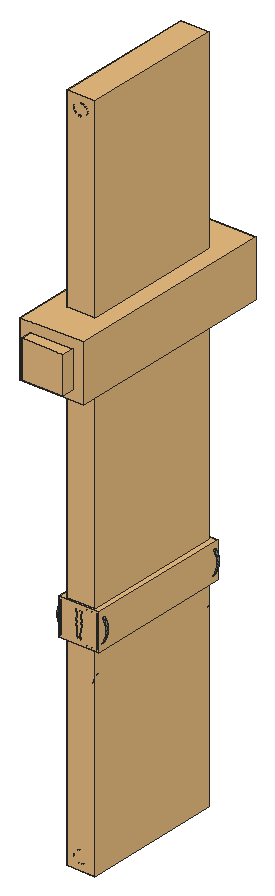
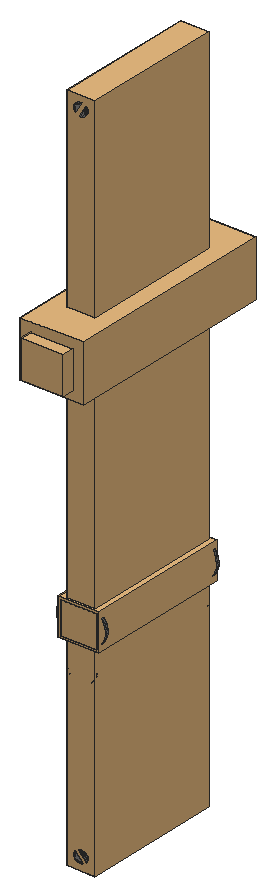
# SketchUp Ruby script. Lengths in inches.
U = 1.inch
M = Sketchup.active_model
def pt(a) = Geom::Point3d.new(a.map { |v| v * U })
def face(e, loops, mat)
  f = e.add_face(loops[0].map { |a| pt(a) })
  loops[1..].each { |l| e.add_face(l.map { |a| pt(a) }).erase! }
  f.material = f.back_material = mat if mat
  f
end
# faces: each face lists its corners as indices into pts; further lists are holes
def faces(e, pts, list, mat = nil) = list.each { |f| face(e, (f[0].is_a?(Array) ? f : [f]).map { |l| l.map { |i| pts[i] } }, mat) }
# xy, xz, yz: faces in a plane at the given z, y or x. An outline is a flat list of corners, or four numbers for a rectangle; further outlines are holes
def ring(l) = l.size == 4 ? [[l[0], l[1]], [l[2], l[1]], [l[2], l[3]], [l[0], l[3]]] : l.each_slice(2).to_a
def flat(e, list, mat, &to3) = list.each { |f| face(e, (f[0].is_a?(Array) ? f : [f]).map { |l| ring(l).map { |u, v| to3.(u, v) } }, mat) }
def xy(e, z, list, mat = nil) = flat(e, list, mat) { |x, y| [x, y, z] }
def xz(e, y, list, mat = nil) = flat(e, list, mat) { |x, z| [x, y, z] }
def yz(e, x, list, mat = nil) = flat(e, list, mat) { |y, z| [x, y, z] }
def lines(e, pts, list) = list.each { |a, b| e.add_line(pt(pts[a]), pt(pts[b])) }
# prism: a flat outline (further loops are holes) pulled along v
def prism(e, loops, v, mat = nil)
  f = face(e, loops, mat); d = Geom::Vector3d.new(v.map { |x| x * U })
  f.pushpull(f.normal.samedirection?(d) ? d.length : -d.length)
end
def box(e, o, s, mat = nil) = prism(e, [[o, [o[0] + s[0], o[1], o[2]], [o[0] + s[0], o[1] + s[1], o[2]], [o[0], o[1] + s[1], o[2]]]], [0, 0, s[2]], mat)
def at(x, y, z, deg = 0) = Geom::Transformation.translation(pt([x, y, z])) * Geom::Transformation.rotation(ORIGIN, Z_AXIS, deg.degrees)
def axes(o, x, y, z) = Geom::Transformation.new([*x, 0, *y, 0, *z, 0, *pt(o).to_a, 1])
def part(name) = M.definitions.add(name)
# library, detail: a bought-in or finely detailed component or shape, given as its bounding box
def library(name, o, s) = part(name).tap { |d| box(d.entities, o, s) }
def detail(e, o, s) = box(e.add_group.entities, o, s)
def put(e, d, t, mat = nil) = e.add_instance(d, t).tap { |i| i.material = mat if mat }
def group(e, t, mat = nil) = e.add_group.tap { |g| g.transformation = t; g.material = mat if mat }.entities
root = M.entities
M.materials.add("Material \#1").color = [140, 140, 140]
c1 = library("3DGeom~14_Defintion",[-102.17,352.37,-727.27],[204.35,204.35,1000])
c2 = library("3DGeom~4_Defintion",[-18.02,-499.97,-221.16],[36.04,1000,262.12])
c3 = part("3DGeom~5_Defintion")
xy(c3.entities,-225.24,[[-0.79,-499.98,-2.33,-499.64,7.45,-496.14],[-0.79,-499.98,7.45,-496.14,1.58,-499.88],[1.58,-499.88,7.45,-496.14,3.84,-499.16],[-2.33,-499.64,7.4,-485.75,7.45,-496.14],[3.84,-499.16,7.45,-496.14,5.85,-497.89],
  [7.45,-496.14,7.4,-485.75,8.24,-487.08],[7.45,-496.14,8.24,-487.08,8.96,-489.34],[7.45,-496.14,8.96,-489.34,9.0625,-491.71],[7.45,-496.14,9.0625,-491.71,8.55,-494.03],[-7.4,-496.08,-8.24,-494.76,2.32,-482.2],
  [-8.24,-494.76,-8.96,-492.5,2.32,-482.2],[-8.96,-492.5,-9.0625,-490.125,2.32,-482.2],[-9.0625,-490.125,-8.55,-487.81,2.32,-482.2],[-8.55,-487.81,-7.45,-485.7,2.32,-482.2],[-7.45,-485.7,-5.85,-483.95,2.32,-482.2],
  [-5.85,-483.95,-3.84,-482.68,2.32,-482.2],[-3.84,-482.68,-1.58,-481.96,2.32,-482.2],[2.32,-482.2,-1.58,-481.96,0.79,-481.86],[0,481.82,-2.35,482.13,-6.92,496.71],[0,481.82,-6.92,496.71,1.55,482.04],
  [-2.35,482.13,-4.55,483.04,-6.92,496.71],[-4.55,483.04,-6.43,484.49,-6.92,496.71],[-6.43,484.49,-7.88,486.37,-6.92,496.71],[6.92,485.12,-1.55,499.8125,7.88,495.47],[6.92,485.12,7.88,495.47,7.88,486.37],
  [-7.88,486.37,-8.79,488.57,-6.92,496.71],[7.88,486.37,7.88,495.47,8.79,488.57],[-8.79,488.57,-9.1,490.92,-6.92,496.71],[8.79,488.57,7.88,495.47,9.1,490.92],[-9.1,490.92,-8.79,493.28,-6.92,496.71],
  [9.1,490.92,7.88,495.47,8.79,493.28],[-8.79,493.28,-7.88,495.47,-6.92,496.71],[7.88,495.47,-1.55,499.8125,0,500.02],[7.88,495.47,0,500.02,2.35,499.71],[7.88,495.47,2.35,499.71,4.55,498.8],
  [7.88,495.47,4.55,498.8,6.43,497.35]],"Material \#1")
xy(c3.entities,-221.57,[[-2.33,-499.64,-5.22,-498.37,7.4,-485.75],[-5.22,-498.37,-7.4,-496.08,5.22,-483.47],[-5.22,-498.37,5.22,-483.47,7.4,-485.75],[-7.4,-496.08,2.32,-482.2,5.22,-483.47],[1.55,482.04,-6.92,496.71,-4.55,498.8],
  [1.55,482.04,-4.55,498.8,4.55,483.04],[4.55,483.04,-4.55,498.8,-1.55,499.8125],[4.55,483.04,-1.55,499.8125,6.92,485.12]],"Material \#1")
xy(c3.entities,38.05,[[-2.33,-499.64,7.4,-485.75,-5.22,-498.37],[-5.22,-498.37,5.22,-483.47,-7.4,-496.08],[-5.22,-498.37,7.4,-485.75,5.22,-483.47],[-7.4,-496.08,5.22,-483.47,2.32,-482.2],[1.55,482.04,-4.55,498.8,-6.92,496.71],
  [1.55,482.04,4.55,483.04,-4.55,498.8],[4.55,483.04,-1.55,499.8125,-4.55,498.8],[4.55,483.04,6.92,485.12,-1.55,499.8125]],"Material \#1")
xy(c3.entities,41.72,[[-0.79,-499.98,7.45,-496.14,-2.33,-499.64],[-0.79,-499.98,1.58,-499.88,7.45,-496.14],[1.58,-499.88,3.84,-499.16,7.45,-496.14],[-2.33,-499.64,7.45,-496.14,7.4,-485.75],[3.84,-499.16,5.85,-497.89,7.45,-496.14],
  [7.45,-496.14,8.24,-487.08,7.4,-485.75],[7.45,-496.14,8.55,-494.03,9.0625,-491.71],[7.45,-496.14,8.96,-489.34,8.24,-487.08],[7.45,-496.14,9.0625,-491.71,8.96,-489.34],[-7.4,-496.08,2.32,-482.2,-8.24,-494.76],
  [-8.24,-494.76,2.32,-482.2,-8.96,-492.5],[-8.96,-492.5,2.32,-482.2,-9.0625,-490.125],[-9.0625,-490.125,2.32,-482.2,-8.55,-487.81],[-8.55,-487.81,2.32,-482.2,-7.45,-485.7],[-7.45,-485.7,2.32,-482.2,-5.85,-483.95],
  [-5.85,-483.95,2.32,-482.2,-3.84,-482.68],[-3.84,-482.68,2.32,-482.2,-1.58,-481.96],[2.32,-482.2,0.79,-481.86,-1.58,-481.96],[0,481.82,-6.92,496.71,-2.35,482.13],[0,481.82,1.55,482.04,-6.92,496.71],
  [-2.35,482.13,-6.92,496.71,-4.55,483.04],[-4.55,483.04,-6.92,496.71,-6.43,484.49],[-6.43,484.49,-6.92,496.71,-7.88,486.37],[6.92,485.12,7.88,495.47,-1.55,499.8125],[6.92,485.12,7.88,486.37,7.88,495.47],
  [-7.88,486.37,-6.92,496.71,-8.79,488.57],[7.88,486.37,8.79,488.57,7.88,495.47],[-8.79,488.57,-6.92,496.71,-9.1,490.92],[8.79,488.57,9.1,490.92,7.88,495.47],[-9.1,490.92,-6.92,496.71,-8.79,493.28],
  [9.1,490.92,8.79,493.28,7.88,495.47],[-8.79,493.28,-6.92,496.71,-7.88,495.47],[7.88,495.47,0,500.02,-1.55,499.8125],[7.88,495.47,2.35,499.71,0,500.02],[7.88,495.47,4.55,498.8,2.35,499.71],
  [7.88,495.47,6.43,497.35,4.55,498.8]],"Material \#1")
c4 = library("3DGeom~1_Defintion",[-60.87,347.29,-704.08],[121.74,121.75,1000])
c5 = part("3DGeom~10_Defintion")
yz(c5.entities,-68.96,[[-797.08,-844.83,-797.08,-827.59,-922.41,-827.59],[-922.41,-844.83,-797.08,-844.83,-922.41,-827.59]],"Material \#1")
yz(c5.entities,68.97,[[-922.41,-844.83,-797.08,-827.59,-797.08,-844.83],[-922.41,-844.83,-922.41,-827.59,-797.08,-827.59],[-797.08,137.93,-922.41,155.17,-797.08,155.17],[-922.41,137.93,-922.41,155.17,-797.08,137.93]],"Material \#1")
p = [[-15.8,-989.55,-844.83],[-15.8,-989.55,-827.59],[0,-991.38,-827.59],[0,-991.38,-844.83],[15.8,-989.55,-827.59],[15.8,-989.55,-844.83],
  [-30.32,-984.36,-844.83],[-30.32,-984.36,-827.59],[30.31,-984.36,-827.59],[30.31,-984.36,-844.83],[-43.12,-976.21,-844.83],[-43.12,-976.21,-827.59],
  [43.12,-976.21,-827.59],[43.12,-976.21,-844.83],[-53.81,-965.53,-844.83],[-53.81,-965.53,-827.59],[53.8,-965.53,-827.59],[53.8,-965.53,-844.83],
  [-61.95,-952.73,-844.83],[-61.95,-952.73,-827.59],[53.8,-965.53,-827.59],[61.95,-952.73,-827.59],[61.95,-952.73,-844.83],[-67.15,-938.21,-844.83],
  [-67.15,-938.21,-827.59],[67.14,-938.21,-827.59],[67.14,-938.21,-844.83],[-68.96,-922.41,-844.83],[-68.96,-922.41,-827.59],[67.14,-938.21,-827.59],
  [68.97,-922.41,-827.59],[68.97,-922.41,-844.83],[-69.1,-794.86,-844.83],[-69.1,-794.86,-827.59],[-68.96,-797.08,-827.59],[-68.96,-797.08,-844.83],
  [68.97,-797.08,-844.83],[68.97,-797.08,-827.59],[69.11,-794.71,-827.59],[69.11,-794.71,-844.83],[-69.48,-792.73,-844.83],[-69.48,-792.73,-827.59],
  [69.53,-792.51,-827.59],[69.53,-792.51,-844.83],[-70.14,-790.6875,-844.83],[-70.14,-790.6875,-827.59],[70.24,-790.48,-827.59],[70.24,-790.48,-844.83],
  [-71.08,-788.73,-844.83],[-71.08,-788.73,-827.59],[71.22,-788.57,-827.59],[71.22,-788.57,-844.83],[-72.32,-786.86,-844.83],[-72.32,-786.86,-827.59],
  [72.47,-786.78,-827.59],[72.47,-786.78,-844.83],[-73.8,-785.17,-844.83],[-73.8,-785.17,-827.59],[74,-785.04,-827.59],[74,-785.04,-844.83],
  [-75.96,-783.21,-844.83],[-75.96,-783.21,-827.59],[74,-785.04,-827.59],[75.76,-783.39,-827.59],[75.76,-783.39,-844.83],[86.625,-772.95,-827.59],
  [86.61,-772.96,-844.83],[-86.89,-773.25,-844.83],[-86.89,-773.25,-827.59],[-75.96,-783.21,-844.83],[-96.66,-761.8,-844.83],[-96.66,-761.8,-827.59],
  [86.625,-772.95,-827.59],[86.63,-772.94,-844.83],[86.61,-772.96,-844.83],[86.625,-772.95,-827.59],[86.62,-772.95,-827.59],[86.62,-772.95,-827.59],
  [96.31,-761.375,-827.59],[96.31,-761.375,-844.83],[86.63,-772.94,-844.83],[86.625,-772.95,-827.59],[86.62,-772.95,-827.59],[-104.96,-749.18,-844.83],
  [-104.96,-749.18,-827.59],[-96.66,-761.8,-827.59],[-96.66,-761.8,-844.83],[96.31,-761.375,-827.59],[104.62,-748.77,-827.59],[104.62,-748.77,-844.83],
  [-111.64,-735.52,-844.83],[-111.64,-735.52,-827.59],[111.39,-735.21,-827.59],[111.39,-735.21,-844.83],[-116.49,-721.23,-844.83],[-116.49,-721.23,-827.59],
  [116.4375,-720.78,-827.59],[116.4375,-720.78,-844.83],[-119.64,-705.62,-844.83],[-119.64,-705.62,-827.59],[119.6,-705.57,-827.59],[119.6,-705.57,-844.83],
  [-120.6875,-689.65,-844.83],[-120.6875,-689.65,-827.59],[120.69,-689.65,-827.59],[120.69,-689.65,-844.83],[-117.5,-662,-844.83],[-117.5,-662,-827.59],
  [117.5,-662,-827.59],[117.5,-662,-844.83],[-108.41,-636.61,-844.83],[-108.41,-636.61,-827.59],[117.5,-662,-844.83],[108.41,-636.61,-827.59],
  [108.41,-636.61,-844.83],[-93.91,-613.95,-844.83],[-93.91,-613.95,-827.59],[-108.41,-636.61,-827.59],[108.41,-636.61,-844.83],[94.16,-614.19,-827.59],
  [94.16,-614.19,-844.83],[94.16,-614.19,-827.59],[75.46,-595.5,-827.59],[75.46,-595.5,-844.83],[-75.46,-595.5,-844.83],[-75.46,-595.5,-827.59],
  [-93.91,-613.95,-827.59],[-93.91,-613.95,-827.59],[-93.91,-613.95,-844.83],[-53.05,-581.24,-844.83],[-53.05,-581.24,-827.59],[-75.46,-595.5,-827.59],
  [-75.46,-595.5,-844.83],[53.05,-581.24,-827.59],[53.05,-581.24,-844.83],[-27.65,-572.16,-844.83],[-27.65,-572.16,-827.59],[-53.05,-581.24,-827.59],
  [-53.05,-581.24,-844.83],[27.66,-572.16,-827.59],[27.66,-572.16,-844.83],[0,-568.97,-844.83],[0,-568.97,-827.59],[-27.65,-572.16,-827.59],
  [-27.65,-572.16,-844.83],[0,-568.97,-844.83],[-15.8,-989.55,155.17],[0,-991.38,155.17],[0,-991.38,137.93],[-15.8,-989.55,137.93],
  [15.8,-989.55,155.17],[15.8,-989.55,137.93],[-30.32,-984.36,155.17],[-30.32,-984.36,137.93],[30.31,-984.36,155.17],[30.31,-984.36,137.93],
  [-43.125,-976.22,155.17],[-43.125,-976.22,137.93],[43.12,-976.22,155.17],[43.12,-976.22,137.93],[-53.81,-965.53,155.17],[-53.81,-965.53,137.93],
  [53.8,-965.53,155.17],[53.8,-965.53,137.93],[-61.96,-952.73,155.17],[-61.95,-952.73,137.93],[61.95,-952.73,155.17],[61.95,-952.73,137.93],
  [53.8,-965.53,137.93],[-67.15,-938.21,155.17],[-67.15,-938.21,137.93],[67.14,-938.21,155.17],[67.14,-938.21,137.93],[-68.96,-922.41,155.17],
  [-68.96,-922.41,137.93],[68.97,-922.41,155.17],[68.97,-922.41,137.93],[67.14,-938.21,137.93],[-68.97,-797.08,155.17],[-68.97,-797.08,137.93],
  [-69.1,-794.86,155.17],[-69.1,-794.86,137.93],[68.97,-797.08,155.17],[69.11,-794.71,155.17],[69.11,-794.71,137.93],[68.97,-797.08,137.93],
  [-69.48,-792.73,155.17],[-69.48,-792.73,137.93],[69.53,-792.51,155.17],[69.53,-792.51,137.93],[-70.14,-790.6875,155.17],[-70.14,-790.6875,137.93],
  [70.24,-790.48,155.17],[70.24,-790.48,137.93],[-71.08,-788.73,155.17],[-71.08,-788.73,137.93],[71.22,-788.57,155.17],[71.22,-788.57,137.93],
  [-72.32,-786.86,155.17],[-72.32,-786.86,137.93],[72.47,-786.78,155.17],[72.47,-786.78,137.93],[-73.8,-785.17,155.17],[-73.8,-785.17,137.93],
  [74,-785.04,155.17],[74,-785.04,137.93],[-75.96,-783.21,155.17],[-75.96,-783.21,137.93],[75.76,-783.39,155.17],[75.76,-783.39,137.93],
  [74,-785.04,137.93],[86.61,-772.96,155.17],[86.625,-772.95,137.93],[-86.88,-773.25,155.17],[-75.96,-783.21,155.17],[-86.88,-773.25,137.93],
  [-96.66,-761.8,155.17],[-96.66,-761.8,137.93],[86.63,-772.94,155.17],[86.625,-772.95,137.93],[86.61,-772.96,155.17],[86.62,-772.95,137.93],
  [86.625,-772.95,137.93],[96.31,-761.375,155.17],[96.31,-761.375,137.93],[86.62,-772.95,137.93],[86.63,-772.94,155.17],[86.62,-772.95,137.93],
  [86.625,-772.95,137.93],[-104.96,-749.18,155.17],[-96.66,-761.8,155.17],[-96.66,-761.8,137.93],[-104.96,-749.18,137.93],[104.62,-748.77,155.17],
  [104.62,-748.77,137.93],[96.31,-761.375,137.93],[-111.64,-735.52,155.17],[-111.64,-735.52,137.93],[111.39,-735.21,155.17],[111.39,-735.21,137.93],
  [-116.49,-721.23,155.17],[-116.49,-721.23,137.93],[116.4375,-720.78,155.17],[116.4375,-720.78,137.93],[-119.64,-705.62,155.17],[-119.64,-705.62,137.93],
  [119.6,-705.57,155.17],[119.6,-705.57,137.93],[-120.6875,-689.65,155.17],[-120.6875,-689.65,137.93],[120.69,-689.65,155.17],[120.69,-689.65,137.93],
  [-117.5,-662,155.17],[-117.5,-662,137.93],[117.5,-662,155.17],[117.5,-662,137.93],[-108.41,-636.61,155.17],[-108.41,-636.61,137.93],
  [117.5,-662,155.17],[108.41,-636.61,155.17],[108.41,-636.61,137.93],[-93.91,-613.95,155.17],[-108.41,-636.61,137.93],[-93.91,-613.95,137.93],
  [108.41,-636.61,155.17],[94.16,-614.19,155.17],[94.16,-614.19,137.93],[75.46,-595.5,155.17],[75.46,-595.5,137.93],[94.16,-614.19,137.93],
  [-75.46,-595.5,155.17],[-93.91,-613.95,155.17],[-93.91,-613.95,137.93],[-75.46,-595.5,137.93],[-53.05,-581.24,155.17],[-75.46,-595.5,155.17],
  [-75.46,-595.5,137.93],[-53.05,-581.24,137.93],[53.05,-581.24,155.17],[53.05,-581.24,137.93],[-27.65,-572.16,155.17],[-53.05,-581.24,155.17],
  [-53.05,-581.24,137.93],[-27.65,-572.16,137.93],[27.65,-572.16,155.17],[27.65,-572.16,137.93],[0,-568.97,155.17],[-27.65,-572.16,155.17],
  [-27.65,-572.16,137.93],[0,-568.97,137.93],[0,-568.97,155.17]]
faces(c5.entities,p,[[0,1,2],[2,3,0],[3,2,4],[4,5,3],[6,7,1],[1,0,6],[5,4,8],[8,9,5],
  [10,11,7],[7,6,10],[9,8,12],[12,13,9],[14,15,11],[11,10,14],[13,12,16],[16,17,13],
  [18,19,15],[15,14,18],[17,20,21],[21,22,17],[23,24,19],[19,18,23],[22,21,25],[25,26,22],
  [27,28,24],[24,23,27],[26,29,30],[30,31,26],[32,33,34],[34,35,32],[36,37,38],[38,39,36],
  [40,41,33],[33,32,40],[39,38,42],[42,43,39],[44,45,41],[41,40,44],[43,42,46],[46,47,43],
  [48,49,45],[45,44,48],[47,46,50],[50,51,47],[52,53,49],[49,48,52],[51,50,54],[54,55,51],
  [56,57,53],[53,52,56],[55,54,58],[58,59,55],[60,61,57],[57,56,60],[59,62,63],[63,64,59],
  [64,63,65],[65,66,64],[67,68,61],[61,69,67],[70,71,68],[68,67,70],[72,73,66],[74,75,76],
  [73,77,78],[78,79,73],[80,81,82],[83,84,85],[85,86,83],[79,87,88],[88,89,79],[90,91,84],
  [84,83,90],[89,88,92],[92,93,89],[94,95,91],[91,90,94],[93,92,96],[96,97,93],[98,99,95],
  [95,94,98],[97,96,100],[100,101,97],[102,103,99],[99,98,102],[101,100,104],[104,105,101],[106,107,103],
  [103,102,106],[105,104,108],[108,109,105],[110,111,107],[107,106,110],[112,108,113],[113,114,112],[115,116,117],
  [117,110,115],[118,113,119],[119,120,118],[120,121,122],[122,123,120],[124,125,126],[127,128,124],[129,130,131],
  [131,132,129],[123,122,133],[133,134,123],[135,136,137],[137,138,135],[134,133,139],[139,140,134],[141,142,143],
  [143,144,141],[140,139,142],[142,145,140],[146,147,148],[148,149,146],[147,150,151],[151,148,147],[152,146,149],
  [149,153,152],[150,154,155],[155,151,150],[156,152,153],[153,157,156],[154,158,159],[159,155,154],[160,156,157],
  [157,161,160],[158,162,163],[163,159,158],[164,160,161],[161,165,164],[162,166,167],[167,168,162],[169,164,165],
  [165,170,169],[166,171,172],[172,167,166],[173,169,170],[170,174,173],[171,175,176],[176,177,171],[178,173,174],
  [174,179,178],[180,178,179],[179,181,180],[182,183,184],[184,185,182],[186,180,181],[181,187,186],[183,188,189],
  [189,184,183],[190,186,187],[187,191,190],[188,192,193],[193,189,188],[194,190,191],[191,195,194],[192,196,197],
  [197,193,192],[198,194,195],[195,199,198],[196,200,201],[201,197,196],[202,198,199],[199,203,202],[200,204,205],
  [205,201,200],[206,202,203],[203,207,206],[204,208,209],[209,210,204],[208,211,212],[212,209,208],[213,214,207],
  [207,215,213],[216,213,215],[215,217,216],[211,218,219],[220,221,222],[218,223,224],[224,225,218],[226,227,228],
  [229,230,231],[231,232,229],[223,233,234],[234,235,223],[236,229,232],[232,237,236],[233,238,239],[239,234,233],
  [240,236,237],[237,241,240],[238,242,243],[243,239,238],[244,240,241],[241,245,244],[242,246,247],[247,243,242],
  [248,244,245],[245,249,248],[246,250,251],[251,247,246],[252,248,249],[249,253,252],[250,254,255],[255,251,250],
  [256,252,253],[253,257,256],[258,259,260],[260,255,258],[261,256,262],[262,263,261],[264,265,266],[266,260,264],
  [265,267,268],[268,269,265],[270,271,272],[272,273,270],[274,275,276],[276,277,274],[267,278,279],[279,268,267],
  [280,281,282],[282,283,280],[278,284,285],[285,279,278],[286,287,288],[288,289,286],[284,290,289],[289,285,284]],"Material \#1")
c6 = library("3DGeom~12_Defintion",[-95.68,-755.75,-830.03],[191.36,191.37,1000])
c7 = library("3DGeom~13_Defintion",[-84.91,-744.98,-830.03],[169.82,169.83,1000])
xy(root,42.551,[[1590.906,529.302,1590.906,529.625,1590.949,529.625],[1590.906,529.302,1590.949,529.625,1590.949,529.302]],"Material \#1")
xy(root,42.907,[[1590.884,529.302,1590.957,529.302,1590.884,529.625],[1590.957,529.302,1590.957,529.625,1590.884,529.625]],"Material \#1")
xz(root,529.625,[[1590.906,42.551,1590.892,42.578,1590.935,42.578],[1590.906,42.551,1590.935,42.578,1590.949,42.551],[1590.892,42.578,1590.884,42.587,1590.943,42.587],[1590.892,42.578,1590.943,42.587,1590.935,42.578],[1590.884,42.587,1590.884,42.607,1590.943,42.607],
  [1590.884,42.587,1590.943,42.607,1590.943,42.587],[1590.884,42.607,1590.892,42.615,1590.935,42.615],[1590.884,42.607,1590.935,42.615,1590.943,42.607],[1590.892,42.615,1590.892,42.649,1590.949,42.649],[1590.892,42.615,1590.949,42.649,1590.935,42.615],
  [1590.892,42.649,1590.892,42.68,1590.949,42.68],[1590.892,42.649,1590.949,42.68,1590.949,42.649],[1590.892,42.68,1590.881,42.705,1590.96,42.705],[1590.892,42.68,1590.96,42.705,1590.949,42.68],[1590.881,42.705,1590.881,42.73,1590.96,42.73],
  [1590.881,42.705,1590.96,42.73,1590.96,42.705],[1590.881,42.73,1590.892,42.756,1590.949,42.756],[1590.881,42.73,1590.949,42.756,1590.96,42.73],[1590.892,42.756,1590.884,42.773,1590.957,42.773],[1590.892,42.756,1590.957,42.773,1590.949,42.756],
  [1590.884,42.773,1590.884,42.831,1590.957,42.831],[1590.884,42.773,1590.957,42.831,1590.957,42.773],[1590.884,42.831,1590.893,42.836,1590.948,42.836],[1590.884,42.831,1590.948,42.836,1590.957,42.831],[1590.893,42.836,1590.893,42.845,1590.948,42.845],
  [1590.893,42.836,1590.948,42.845,1590.948,42.836],[1590.893,42.845,1590.884,42.849,1590.957,42.849],[1590.893,42.845,1590.957,42.849,1590.948,42.845],[1590.884,42.849,1590.884,42.907,1590.957,42.907],[1590.884,42.849,1590.957,42.907,1590.957,42.849]],"Material \#1")
xz(root,529.66,[[1590.92,41.959,1590.837,41.976,1590.877,41.963],[1590.92,41.959,1591.004,41.976,1590.837,41.976],[1590.92,41.959,1590.964,41.963,1591.004,41.976],[1590.837,41.976,1590.73,42.452,1590.735,42.089],[1590.837,41.976,1591.105,42.089,1590.73,42.452],
  [1590.837,41.976,1590.735,42.089,1590.772,42.022],[1590.837,41.976,1590.772,42.022,1590.801,41.996],[1590.837,41.976,1591.004,41.976,1591.105,42.089],[1591.004,41.976,1591.039,41.996,1591.068,42.022],[1590.772,42.022,1590.735,42.089,1590.749,42.054],
  [1591.105,42.089,1590.723,42.477,1590.726,42.471],[1591.105,42.089,1591.11,42.128,1590.723,42.477],[1591.105,42.089,1590.726,42.471,1590.728,42.465],[1591.105,42.089,1590.728,42.465,1590.73,42.459],[1590.735,42.089,1590.73,42.452,1590.73,42.128],
  [1591.105,42.089,1590.73,42.459,1590.73,42.452],[1591.11,42.128,1590.686,42.562,1590.723,42.477],[1591.11,42.128,1590.733,42.521,1590.686,42.562],[1591.11,42.128,1590.788,42.489,1590.733,42.521],[1591.11,42.128,1590.851,42.469,1590.788,42.489],
  [1591.11,42.128,1590.92,42.462,1590.851,42.469],[1591.11,42.128,1590.989,42.469,1590.92,42.462],[1590.655,42.918,1590.733,42.9375,1590.788,42.969],[1590.655,42.918,1590.788,42.969,1590.92,43.032],[1590.655,42.918,1590.92,43.032,1590.771,43.001],
  [1591.185,42.918,1590.92,43.032,1591.052,42.969],[1590.788,42.969,1590.851,42.989,1590.92,43.032],[1591.052,42.969,1590.92,43.032,1590.989,42.989],[1590.851,42.989,1590.92,42.996,1590.92,43.032],[1590.989,42.989,1590.92,43.032,1590.92,42.996],
  [1590.771,43.001,1590.92,43.032,1590.842,43.024],[1591.07,43.001,1590.998,43.024,1590.92,43.032]],"Material \#1")
xz(root,531.048,[[1591.185,42.918,1591.052,42.969,1590.92,43.032],[1591.052,42.969,1590.989,42.989,1590.92,43.032],[1590.989,42.989,1590.92,42.996,1590.92,43.032],[1591.07,43.001,1590.92,43.032,1590.998,43.024]],"Material \#1")
yz(root,1590.884,[[529.625,42.849,529.302,42.907,529.625,42.907]],"Material \#1")
yz(root,1590.892,[[529.625,42.615,529.302,42.649,529.625,42.649]],"Material \#1")
yz(root,1590.949,[[529.302,42.649,529.625,42.649,529.625,42.68],[529.302,42.649,529.625,42.68,529.302,42.68]],"Material \#1")
yz(root,1590.957,[[529.302,42.773,529.625,42.773,529.625,42.831]],"Material \#1")
yz(root,1590.96,[[529.302,42.705,529.625,42.705,529.625,42.73],[529.302,42.705,529.625,42.73,529.302,42.73]],"Material \#1")
p = [[1590.892,529.625,42.615],[1590.888,529.302,42.611],[1590.892,529.302,42.649],[1590.892,529.625,42.649],[1590.892,529.302,42.649],[1590.886,529.302,42.693],
  [1590.949,529.625,42.649],[1590.949,529.302,42.649],[1590.939,529.302,42.611],[1590.935,529.625,42.578],[1590.939,529.302,42.582],[1590.949,529.302,42.551],
  [1590.888,529.302,42.611],[1590.884,529.625,42.607],[1590.884,529.625,42.587],[1590.888,529.302,42.582],[1590.939,529.302,42.582],[1590.943,529.625,42.587],
  [1590.943,529.625,42.607],[1590.939,529.302,42.611],[1590.888,529.302,42.611],[1590.892,529.625,42.615],[1590.884,529.625,42.607],[1590.888,529.302,42.582],
  [1590.884,529.625,42.587],[1590.892,529.625,42.578],[1590.886,529.302,42.693],[1590.892,529.625,42.68],[1590.892,529.625,42.649],[1590.939,529.302,42.611],
  [1590.935,529.625,42.615],[1590.949,529.625,42.649],[1590.939,529.302,42.611],[1590.943,529.625,42.607],[1590.935,529.625,42.615],[1590.939,529.302,42.582],
  [1590.935,529.625,42.578],[1590.943,529.625,42.587],[1590.949,529.302,42.551],[1590.949,529.625,42.551],[1590.935,529.625,42.578],[1590.888,529.302,42.582],
  [1590.892,529.625,42.578],[1590.906,529.625,42.551],[1590.906,529.302,42.551],[1590.888,529.302,42.582],[1590.892,529.625,42.68],[1590.886,529.302,42.693],
  [1590.881,529.302,42.718],[1590.881,529.625,42.705],[1590.881,529.302,42.718],[1590.886,529.302,42.743],[1590.949,529.625,42.756],[1590.949,529.302,42.756],
  [1590.96,529.302,42.73],[1590.96,529.625,42.705],[1590.96,529.302,42.705],[1590.949,529.302,42.68],[1590.881,529.625,42.73],[1590.886,529.302,42.743],
  [1590.888,529.302,42.765],[1590.881,529.302,42.718],[1590.881,529.625,42.705],[1590.892,529.625,42.68],[1590.96,529.302,42.73],[1590.96,529.625,42.73],
  [1590.949,529.625,42.756],[1590.949,529.302,42.68],[1590.949,529.625,42.68],[1590.96,529.625,42.705],[1590.888,529.302,42.765],[1590.892,529.625,42.756],
  [1590.881,529.625,42.73],[1590.886,529.302,42.743],[1590.881,529.625,42.73],[1590.881,529.625,42.705],[1590.957,529.625,42.773],[1590.957,529.302,42.773],
  [1590.949,529.302,42.756],[1590.884,529.625,42.849],[1590.888,529.302,42.836],[1590.884,529.302,42.907],[1590.884,529.625,42.773],[1590.885,529.302,42.777],
  [1590.888,529.302,42.836],[1590.892,529.625,42.756],[1590.888,529.302,42.765],[1590.885,529.302,42.777],[1590.949,529.302,42.756],[1590.949,529.625,42.756],
  [1590.957,529.625,42.773],[1590.888,529.302,42.836],[1590.884,529.625,42.831],[1590.884,529.625,42.773],[1590.885,529.302,42.777],[1590.884,529.625,42.773],
  [1590.892,529.625,42.756],[1590.953,529.302,42.842],[1590.957,529.625,42.831],[1590.948,529.625,42.836],[1590.888,529.302,42.836],[1590.893,529.625,42.845],
  [1590.893,529.625,42.836],[1590.888,529.302,42.836],[1590.884,529.625,42.849],[1590.888,529.302,42.836],[1590.884,529.625,42.831],[1590.953,529.302,42.842],
  [1590.948,529.625,42.845],[1590.957,529.625,42.849],[1590.953,529.302,42.842],[1590.957,529.625,42.907],[1590.957,529.302,42.907],[1590.953,529.302,42.842],
  [1590.957,529.625,42.831],[1590.953,529.302,42.842],[1590.957,529.302,42.773],[1590.953,529.302,42.842],[1590.957,529.625,42.849],[1590.957,529.625,42.907]]
faces(root,p,[[0,1,2],[3,4,5],[6,7,8],[9,10,11],[12,13,14],[14,15,12],[16,17,18],[18,19,16],
  [20,21,22],[23,24,25],[26,27,28],[29,30,31],[32,33,34],[35,36,37],[38,39,40],[41,42,43],
  [43,44,45],[46,47,48],[49,50,51],[52,53,54],[55,56,57],[58,59,60],[61,62,63],[64,65,66],
  [67,68,69],[70,71,72],[73,74,75],[76,77,78],[79,80,81],[82,83,84],[85,86,87],[88,89,90],
  [91,92,93],[94,95,96],[97,98,99],[100,101,102],[103,104,101],[105,102,106],[107,108,109],[110,99,108],
  [111,112,113],[114,115,116],[117,118,119]],"Material \#1")
put(root,c1,axes([1590.92,531.05,44.51],[0.0044,0,0],[0,0,0.00392],[0,0.00306,0]),"Material \#1")
put(root,c2,axes([1590.92,531.05,44.51],[0.0111,0,0],[0,0,0.00988],[0,0.00771,0]),"Material \#1")
put(root,c3,axes([1590.92,531.05,44.51],[0.0109,0,0],[0,0,0.0097],[0,0.00757,0]),"Material \#1")
put(root,c4,axes([1590.92,531.05,44.51],[0.0049,0,0],[0,0,0.00436],[0,0.0034,0]),"Material \#1")
put(root,c5,axes([1590.92,531.05,44.51],[0.0029,0,0],[0,0,0.00258],[0,0.00201,0]),"Material \#1")
put(root,c6,axes([1590.92,531.05,44.51],[0.00303,0,0],[0,0,0.0027],[0,0.0021,0]),"Material \#1")
put(root,c7,axes([1590.92,531.05,44.51],[0.00303,0,0],[0,0,0.0027],[0,0.0021,0]),"Material \#1")
